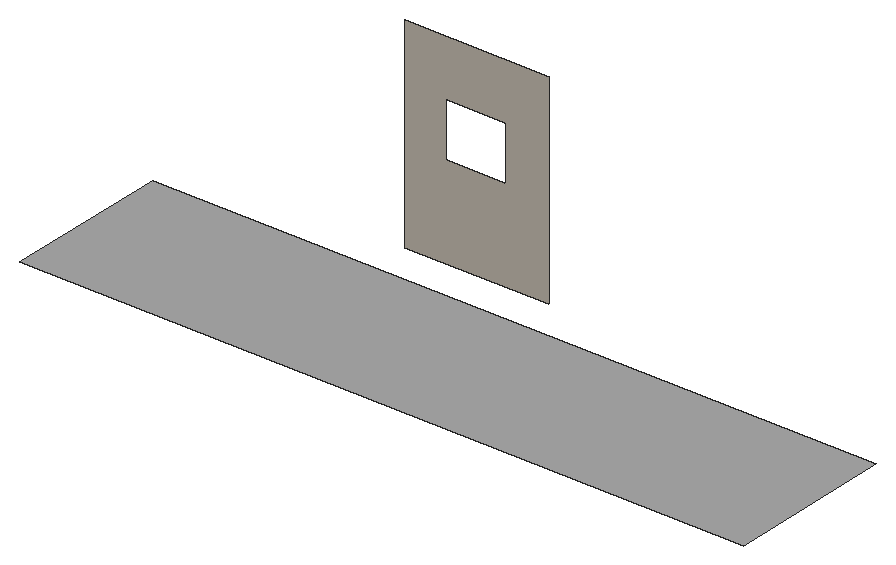
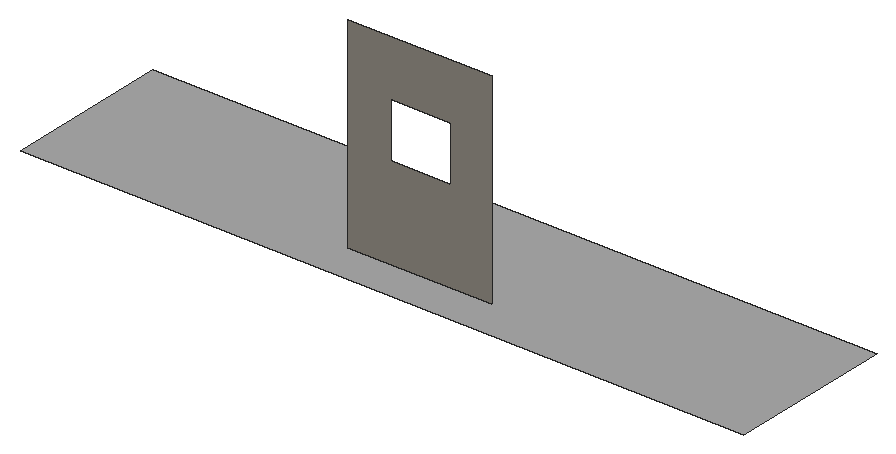
# SketchUp Ruby script. Lengths in inches.
U = 1.inch
M = Sketchup.active_model
def pt(a) = Geom::Point3d.new(a.map { |v| v * U })
def face(e, loops, mat)
  f = e.add_face(loops[0].map { |a| pt(a) })
  loops[1..].each { |l| e.add_face(l.map { |a| pt(a) }).erase! }
  f.material = f.back_material = mat if mat
  f
end
# faces: each face lists its corners as indices into pts; further lists are holes
def faces(e, pts, list, mat = nil) = list.each { |f| face(e, (f[0].is_a?(Array) ? f : [f]).map { |l| l.map { |i| pts[i] } }, mat) }
# xy, xz, yz: faces in a plane at the given z, y or x. An outline is a flat list of corners, or four numbers for a rectangle; further outlines are holes
def ring(l) = l.size == 4 ? [[l[0], l[1]], [l[2], l[1]], [l[2], l[3]], [l[0], l[3]]] : l.each_slice(2).to_a
def flat(e, list, mat, &to3) = list.each { |f| face(e, (f[0].is_a?(Array) ? f : [f]).map { |l| ring(l).map { |u, v| to3.(u, v) } }, mat) }
def xy(e, z, list, mat = nil) = flat(e, list, mat) { |x, y| [x, y, z] }
def xz(e, y, list, mat = nil) = flat(e, list, mat) { |x, z| [x, y, z] }
def yz(e, x, list, mat = nil) = flat(e, list, mat) { |y, z| [x, y, z] }
def lines(e, pts, list) = list.each { |a, b| e.add_line(pt(pts[a]), pt(pts[b])) }
# prism: a flat outline (further loops are holes) pulled along v
def prism(e, loops, v, mat = nil)
  f = face(e, loops, mat); d = Geom::Vector3d.new(v.map { |x| x * U })
  f.pushpull(f.normal.samedirection?(d) ? d.length : -d.length)
end
def box(e, o, s, mat = nil) = prism(e, [[o, [o[0] + s[0], o[1], o[2]], [o[0] + s[0], o[1] + s[1], o[2]], [o[0], o[1] + s[1], o[2]]]], [0, 0, s[2]], mat)
def at(x, y, z, deg = 0) = Geom::Transformation.translation(pt([x, y, z])) * Geom::Transformation.rotation(ORIGIN, Z_AXIS, deg.degrees)
def axes(o, x, y, z) = Geom::Transformation.new([*x, 0, *y, 0, *z, 0, *pt(o).to_a, 1])
def part(name) = M.definitions.add(name)
# library, detail: a bought-in or finely detailed component or shape, given as its bounding box
def library(name, o, s) = part(name).tap { |d| box(d.entities, o, s) }
def detail(e, o, s) = box(e.add_group.entities, o, s)
def put(e, d, t, mat = nil) = e.add_instance(d, t).tap { |i| i.material = mat if mat }
def group(e, t, mat = nil) = e.add_group.tap { |g| g.transformation = t; g.material = mat if mat }.entities
root = M.entities
M.materials.add("[Color M03]").color = [170, 170, 170]
M.materials.add("[Stone Masonry Multi]").color = [182, 175, 164]
xy(root,137.875,[[176.75,197.29,298.6,225.17]],"[Color M03]")
xz(root,225.17,[[[219.28,142.6875,243.46,177],[226.04,158.26,236.29,167.57]]],"[Stone Masonry Multi]")
